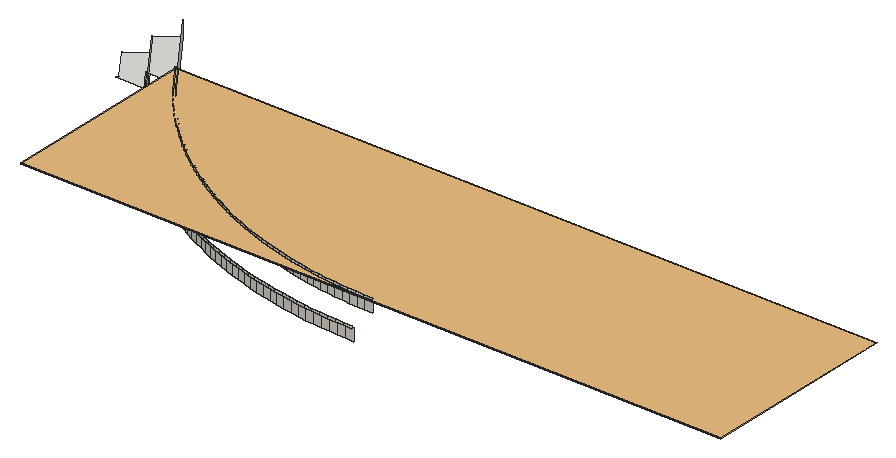
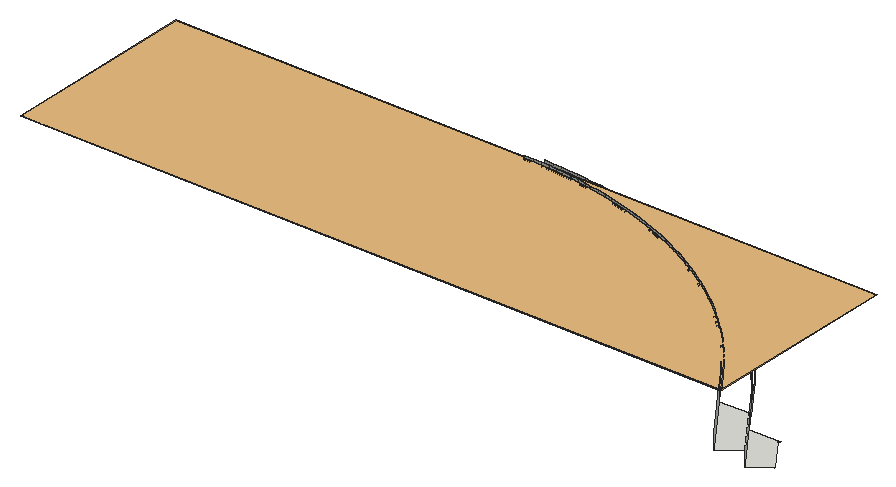
# SketchUp Ruby script. Lengths in inches.
U = 1.inch
M = Sketchup.active_model
def pt(a) = Geom::Point3d.new(a.map { |v| v * U })
def face(e, loops, mat)
  f = e.add_face(loops[0].map { |a| pt(a) })
  loops[1..].each { |l| e.add_face(l.map { |a| pt(a) }).erase! }
  f.material = f.back_material = mat if mat
  f
end
# faces: each face lists its corners as indices into pts; further lists are holes
def faces(e, pts, list, mat = nil) = list.each { |f| face(e, (f[0].is_a?(Array) ? f : [f]).map { |l| l.map { |i| pts[i] } }, mat) }
# xy, xz, yz: faces in a plane at the given z, y or x. An outline is a flat list of corners, or four numbers for a rectangle; further outlines are holes
def ring(l) = l.size == 4 ? [[l[0], l[1]], [l[2], l[1]], [l[2], l[3]], [l[0], l[3]]] : l.each_slice(2).to_a
def flat(e, list, mat, &to3) = list.each { |f| face(e, (f[0].is_a?(Array) ? f : [f]).map { |l| ring(l).map { |u, v| to3.(u, v) } }, mat) }
def xy(e, z, list, mat = nil) = flat(e, list, mat) { |x, y| [x, y, z] }
def xz(e, y, list, mat = nil) = flat(e, list, mat) { |x, z| [x, y, z] }
def yz(e, x, list, mat = nil) = flat(e, list, mat) { |y, z| [x, y, z] }
def lines(e, pts, list) = list.each { |a, b| e.add_line(pt(pts[a]), pt(pts[b])) }
# prism: a flat outline (further loops are holes) pulled along v
def prism(e, loops, v, mat = nil)
  f = face(e, loops, mat); d = Geom::Vector3d.new(v.map { |x| x * U })
  f.pushpull(f.normal.samedirection?(d) ? d.length : -d.length)
end
def box(e, o, s, mat = nil) = prism(e, [[o, [o[0] + s[0], o[1], o[2]], [o[0] + s[0], o[1] + s[1], o[2]], [o[0], o[1] + s[1], o[2]]]], [0, 0, s[2]], mat)
def at(x, y, z, deg = 0) = Geom::Transformation.translation(pt([x, y, z])) * Geom::Transformation.rotation(ORIGIN, Z_AXIS, deg.degrees)
def axes(o, x, y, z) = Geom::Transformation.new([*x, 0, *y, 0, *z, 0, *pt(o).to_a, 1])
def part(name) = M.definitions.add(name)
# library, detail: a bought-in or finely detailed component or shape, given as its bounding box
def library(name, o, s) = part(name).tap { |d| box(d.entities, o, s) }
def detail(e, o, s) = box(e.add_group.entities, o, s)
def put(e, d, t, mat = nil) = e.add_instance(d, t).tap { |i| i.material = mat if mat }
def group(e, t, mat = nil) = e.add_group.tap { |g| g.transformation = t; g.material = mat if mat }.entities
root = M.entities
M.materials.add("Arta-Ceramic-Moonstone-White-24x24-4K").color = [209, 205, 196]
c1 = library("Mesh Light\#5",[-0.5,-0.5,-0.1],[1,1,0.2])
xy(root,18,[[859.84,194.875,871.84,194.875,857.89,214.375,849.96,208.69,859.5,195.35]])
xy(root,18,[[858.84,194.875,859.84,194.875,859.5,195.35]],"Arta-Ceramic-Moonstone-White-24x24-4K")
xy(root,23,[[870.84,194.875,870.78,194.96,871.44,195.43,871.84,194.875]],"Arta-Ceramic-Moonstone-White-24x24-4K")
xy(root,24,[[871.84,194.875,883.84,194.875,865.83,220.05,857.89,214.375,871.44,195.43]])
xy(root,24,[[870.84,194.875,871.84,194.875,871.44,195.43,870.78,194.96]],"Arta-Ceramic-Moonstone-White-24x24-4K")
xy(root,29,[[882.84,194.875,882.57,195.26,883.23,195.73,883.84,194.875]],"Arta-Ceramic-Moonstone-White-24x24-4K")
p = [[1020.9,108.58,23],[1020.9,108.58,18],[1024.28,108.54,18],[1024.28,108.54,23],[1017.51,108.67,23],[1017.51,108.67,18],
  [1014.13,108.84,23],[1014.13,108.84,18],[1010.76,109.0625,23],[1010.76,109.0625,18],[1007.39,109.35,23],[1007.39,109.35,18],
  [1004.02,109.71,23],[1004.02,109.71,18],[1000.66,110.13,23],[1000.66,110.13,18],[997.3125,110.62,23],[997.3125,110.62,18],
  [993.97,111.17,23],[993.97,111.17,18],[990.65,111.78,23],[990.65,111.78,18],[987.33,112.46,23],[987.33,112.46,18],
  [984.03,113.2,23],[984.03,113.2,18],[980.74,114,23],[980.74,114,18],[977.47,114.87,23],[977.47,114.87,18],
  [974.22,115.8,23],[974.22,115.8,18],[970.98,116.79,23],[970.98,116.79,18],[967.77,117.84,23],[967.77,117.84,18],
  [964.57,118.96,23],[964.57,118.96,18],[961.4,120.13,23],[961.4,120.13,18],[958.25,121.37,23],[958.25,121.37,18],
  [955.12,122.67,23],[955.12,122.67,18],[952.02,124.02,23],[952.02,124.02,18],[948.95,125.44,23],[948.95,125.44,18],
  [945.9,126.92,23],[945.9,126.92,18],[942.88,128.45,23],[942.88,128.45,18],[939.9,130.04,23],[939.9,130.04,18],
  [936.94,131.6875,23],[936.94,131.6875,18],[934.02,133.39,23],[934.02,133.39,18],[931.13,135.15,23],[931.13,135.15,18],
  [928.27,136.96,23],[928.27,136.96,18],[925.45,138.83,23],[925.45,138.83,18],[922.67,140.76,23],[922.67,140.76,18],
  [919.92,142.73,23],[919.92,142.73,18],[917.21,144.76,23],[917.21,144.76,18],[914.54,146.84,23],[914.54,146.84,18],
  [911.91,148.97,23],[911.91,148.97,18],[909.32,151.15,23],[909.32,151.15,18],[906.78,153.38,23],[906.78,153.38,18],
  [904.28,155.66,23],[904.28,155.66,18],[901.82,157.99,23],[901.82,157.99,18],[899.41,160.36,23],[899.41,160.36,18],
  [897.04,162.78,23],[897.04,162.78,18],[894.72,165.24,23],[894.72,165.24,18],[892.45,167.75,23],[892.45,167.75,18],
  [890.22,170.3,23],[890.22,170.3,18],[888.05,172.89,23],[888.05,172.89,18],[885.92,175.53,23],[885.92,175.53,18],
  [883.85,178.2,23],[883.85,178.2,18],[881.83,180.92,23],[881.83,180.92,18],[871.84,194.875,23],[871.84,194.875,18],
  [857.89,214.375,18],[871.44,195.43,23],[871.44,195.43,24],[857.89,214.375,24],[1020.88,107.76,24],[1020.88,107.76,23],
  [1024.28,107.73,23],[1024.28,107.73,24],[1017.48,107.86,24],[1017.48,107.86,23],[1014.09,108.02,24],[1014.09,108.02,23],
  [1010.7,108.25,24],[1010.7,108.25,23],[1007.31,108.54,24],[1007.31,108.54,23],[1003.93,108.9,24],[1003.93,108.9,23],
  [1000.55,109.33,24],[1000.55,109.33,23],[997.19,109.8125,24],[997.19,109.8125,23],[993.84,110.37,24],[993.84,110.37,23],
  [990.49,110.98,24],[990.49,110.98,23],[987.16,111.66,24],[987.16,111.66,23],[983.84,112.41,24],[983.84,112.41,23],
  [980.54,113.21,24],[980.54,113.21,23],[977.25,114.08,24],[977.25,114.08,23],[973.99,115.02,24],[973.99,115.02,23],
  [970.74,116.01,24],[970.74,116.01,23],[967.5,117.07,24],[967.5,117.07,23],[964.29,118.19,24],[964.29,118.19,23],
  [961.11,119.375,24],[961.11,119.375,23],[957.94,120.62,24],[957.94,120.62,23],[954.8,121.92,24],[954.8,121.92,23],
  [951.6875,123.28,24],[951.6875,123.28,23],[948.6,124.71,24],[948.6,124.71,23],[945.54,126.1875,24],[945.54,126.1875,23],
  [942.51,127.73,24],[942.51,127.73,23],[939.51,129.32,24],[939.51,129.32,23],[936.54,130.98,24],[936.54,130.98,23],
  [933.6,132.69,24],[933.6,132.69,23],[930.7,134.46,24],[930.7,134.46,23],[927.83,136.28,24],[927.83,136.28,23],
  [924.99,138.16,24],[924.99,138.16,23],[922.2,140.09,24],[922.2,140.09,23],[919.4375,142.08,24],[919.4375,142.08,23],
  [916.72,144.11,24],[916.72,144.11,23],[914.03,146.2,24],[914.03,146.2,23],[911.39,148.34,24],[911.39,148.34,23],
  [908.79,150.54,24],[908.79,150.54,23],[906.24,152.78,24],[906.24,152.78,23],[903.72,155.07,24],[903.72,155.07,23],
  [901.25,157.4,24],[901.25,157.4,23],[898.83,159.79,24],[898.83,159.79,23],[896.45,162.22,24],[896.45,162.22,23],
  [894.12,164.69,24],[894.12,164.69,23],[891.84,167.21,24],[891.84,167.21,23],[889.61,169.77,24],[889.61,169.77,23],
  [887.42,172.38,24],[887.42,172.38,23],[885.29,175.02,24],[885.29,175.02,23],[883.2,177.71,24],[883.2,177.71,23],
  [881.17,180.4375,24],[881.17,180.4375,23],[870.84,194.875,24],[870.84,194.875,23],[870.78,194.96,23],[870.78,194.96,24],
  [1017.89,118.43,29],[1017.89,118.43,24],[1021.08,118.33,24],[1021.08,118.33,29],[1024.28,118.3,24],[1024.28,118.3,29],
  [1014.7,118.58,29],[1014.7,118.58,24],[1011.51,118.79,29],[1011.51,118.79,24],[1008.32,119.07,29],[1008.32,119.07,24],
  [1005.14,119.41,29],[1005.14,119.41,24],[1001.97,119.8,29],[1001.97,119.8,24],[998.81,120.26,29],[998.81,120.26,24],
  [995.65,120.78,29],[995.65,120.78,24],[992.51,121.36,29],[992.51,121.36,24],[989.375,122,29],[989.375,122,24],
  [986.26,122.7,29],[986.26,122.7,24],[983.15,123.46,29],[983.15,123.46,24],[980.0625,124.28,29],[980.0625,124.28,24],
  [976.99,125.16,29],[976.99,125.16,24],[973.93,126.09,29],[973.93,126.09,24],[970.89,127.09,29],[970.89,127.09,24],
  [967.875,128.14,29],[967.875,128.14,24],[964.875,129.25,29],[964.875,129.25,24],[961.9,130.42,29],[961.9,130.42,24],
  [958.95,131.65,29],[958.95,131.65,24],[956.02,132.93,29],[956.02,132.93,24],[953.12,134.27,29],[953.12,134.27,24],
  [950.24,135.66,29],[950.24,135.66,24],[947.39,137.11,29],[947.39,137.11,24],[944.57,138.61,29],[944.57,138.61,24],
  [941.77,140.16,29],[941.77,140.16,24],[939.01,141.77,29],[939.01,141.77,24],[936.28,143.4375,29],[936.28,143.4375,24],
  [933.58,145.15,29],[933.58,145.15,24],[930.92,146.92,29],[930.92,146.92,24],[928.29,148.73,29],[928.29,148.73,24],
  [925.69,150.6,29],[925.69,150.6,24],[923.13,152.52,29],[923.13,152.52,24],[920.61,154.48,29],[920.61,154.48,24],
  [918.13,156.49,29],[918.13,156.49,24],[915.68,158.55,29],[915.68,158.55,24],[913.28,160.66,29],[913.28,160.66,24],
  [910.92,162.8125,29],[910.92,162.8125,24],[908.59,165.01,29],[908.59,165.01,24],[906.32,167.25,29],[906.32,167.25,24],
  [904.08,169.54,29],[904.08,169.54,24],[901.89,171.87,29],[901.89,171.87,24],[899.74,174.23,29],[899.74,174.23,24],
  [897.64,176.64,29],[897.64,176.64,24],[895.59,179.09,29],[895.59,179.09,24],[893.58,181.58,29],[893.58,181.58,24],
  [891.62,184.11,29],[891.62,184.11,24],[889.71,186.67,29],[889.71,186.67,24],[883.84,194.875,29],[883.84,194.875,24],
  [865.83,220.05,24],[883.23,195.73,29],[883.23,195.73,30],[865.83,220.05,30],[1017.86,117.61,30],[1017.86,117.61,29],
  [1021.07,117.52,29],[1021.07,117.52,30],[1024.28,117.49,29],[1024.28,117.49,30],[1014.65,117.77,30],[1014.65,117.77,29],
  [1011.44,117.98,30],[1011.44,117.98,29],[1008.24,118.26,30],[1008.24,118.26,29],[1005.05,118.6,30],[1005.05,118.6,29],
  [1001.86,119,30],[1001.86,119,29],[998.68,119.46,30],[998.68,119.46,29],[995.51,119.98,30],[995.51,119.98,29],
  [992.35,120.5625,30],[992.35,120.5625,29],[989.21,121.2,30],[989.21,121.2,29],[986.07,121.91,30],[986.07,121.91,29],
  [982.95,122.67,30],[982.95,122.67,29],[979.85,123.49,30],[979.85,123.49,29],[976.76,124.375,30],[976.76,124.375,29],
  [973.68,125.32,30],[973.68,125.32,29],[970.63,126.32,30],[970.63,126.32,29],[967.6,127.375,30],[967.6,127.375,29],
  [964.59,128.49,30],[964.59,128.49,29],[961.6,129.67,30],[961.6,129.67,29],[958.63,130.9,30],[958.63,130.9,29],
  [955.6875,132.1875,30],[955.6875,132.1875,29],[952.77,133.53,30],[952.77,133.53,29],[949.88,134.93,30],[949.88,134.93,29],
  [947.01,136.38,30],[947.01,136.38,29],[944.18,137.89,30],[944.18,137.89,29],[941.37,139.46,30],[941.37,139.46,29],
  [938.6,141.08,30],[938.6,141.08,29],[935.85,142.75,30],[935.85,142.75,29],[933.14,144.47,30],[933.14,144.47,29],
  [930.46,146.24,30],[930.46,146.24,29],[927.82,148.07,30],[927.82,148.07,29],[925.21,149.94,30],[925.21,149.94,29],
  [922.64,151.87,30],[922.64,151.87,29],[920.11,153.84,30],[920.11,153.84,29],[917.61,155.87,30],[917.61,155.87,29],
  [915.15,157.9375,30],[915.15,157.9375,29],[912.74,160.05,30],[912.74,160.05,29],[910.36,162.22,30],[910.36,162.22,29],
  [908.03,164.43,30],[908.03,164.43,29],[905.74,166.68,30],[905.74,166.68,29],[903.49,168.97,30],[903.49,168.97,29],
  [901.29,171.3125,30],[901.29,171.3125,29],[899.13,173.69,30],[899.13,173.69,29],[897.02,176.12,30],[897.02,176.12,29],
  [894.96,178.58,30],[894.96,178.58,29],[892.94,181.08,30],[892.94,181.08,29],[890.97,183.62,30],[890.97,183.62,29],
  [889.06,186.19,30],[889.06,186.19,29],[882.84,194.875,30],[882.84,194.875,29],[882.57,195.26,29],[882.57,195.26,30]]
faces(root,p,[[0,1,2,3],[4,5,1,0],[6,7,5,4],[8,9,7,6],[10,11,9,8],[12,13,11,10],[14,15,13,12],[16,17,15,14],
  [18,19,17,16],[20,21,19,18],[22,23,21,20],[24,25,23,22],[26,27,25,24],[28,29,27,26],[30,31,29,28],[32,33,31,30],
  [34,35,33,32],[36,37,35,34],[38,39,37,36],[40,41,39,38],[42,43,41,40],[44,45,43,42],[46,47,45,44],[48,49,47,46],
  [50,51,49,48],[52,53,51,50],[54,55,53,52],[56,57,55,54],[58,59,57,56],[60,61,59,58],[62,63,61,60],[64,65,63,62],
  [66,67,65,64],[68,69,67,66],[70,71,69,68],[72,73,71,70],[74,75,73,72],[76,77,75,74],[78,79,77,76],[80,81,79,78],
  [82,83,81,80],[84,85,83,82],[86,87,85,84],[88,89,87,86],[90,91,89,88],[92,93,91,90],[94,95,93,92],[96,97,95,94],
  [98,99,97,96],[100,101,99,98],[106,107,108,109],[110,111,107,106],[112,113,111,110],[114,115,113,112],[116,117,115,114],[118,119,117,116],
  [120,121,119,118],[122,123,121,120],[124,125,123,122],[126,127,125,124],[128,129,127,126],[130,131,129,128],[132,133,131,130],[134,135,133,132],
  [136,137,135,134],[138,139,137,136],[140,141,139,138],[142,143,141,140],[144,145,143,142],[146,147,145,144],[148,149,147,146],[150,151,149,148],
  [152,153,151,150],[154,155,153,152],[156,157,155,154],[158,159,157,156],[160,161,159,158],[162,163,161,160],[164,165,163,162],[166,167,165,164],
  [168,169,167,166],[170,171,169,168],[172,173,171,170],[174,175,173,172],[176,177,175,174],[178,179,177,176],[180,181,179,178],[182,183,181,180],
  [184,185,183,182],[186,187,185,184],[188,189,187,186],[190,191,189,188],[192,193,191,190],[194,195,193,192],[196,197,195,194],[198,199,197,196],
  [200,201,199,198],[202,203,201,200],[204,205,203,202],[204,206,207,205],[208,207,206,209],[103,208,209,104],[210,211,212,213],[213,212,214,215],
  [216,217,211,210],[218,219,217,216],[220,221,219,218],[222,223,221,220],[224,225,223,222],[226,227,225,224],[228,229,227,226],[230,231,229,228],
  [232,233,231,230],[234,235,233,232],[236,237,235,234],[238,239,237,236],[240,241,239,238],[242,243,241,240],[244,245,243,242],[246,247,245,244],
  [248,249,247,246],[250,251,249,248],[252,253,251,250],[254,255,253,252],[256,257,255,254],[258,259,257,256],[260,261,259,258],[262,263,261,260],
  [264,265,263,262],[266,267,265,264],[268,269,267,266],[270,271,269,268],[272,273,271,270],[274,275,273,272],[276,277,275,274],[278,279,277,276],
  [280,281,279,278],[282,283,281,280],[284,285,283,282],[286,287,285,284],[288,289,287,286],[290,291,289,288],[292,293,291,290],[294,295,293,292],
  [296,297,295,294],[298,299,297,296],[300,301,299,298],[302,303,301,300],[304,305,303,302],[306,307,305,304],[308,309,307,306],[310,311,309,308],
  [316,317,318,319],[319,318,320,321],[322,323,317,316],[324,325,323,322],[326,327,325,324],[328,329,327,326],[330,331,329,328],[332,333,331,330],
  [334,335,333,332],[336,337,335,334],[338,339,337,336],[340,341,339,338],[342,343,341,340],[344,345,343,342],[346,347,345,344],[348,349,347,346],
  [350,351,349,348],[352,353,351,350],[354,355,353,352],[356,357,355,354],[358,359,357,356],[360,361,359,358],[362,363,361,360],[364,365,363,362],
  [366,367,365,364],[368,369,367,366],[370,371,369,368],[372,373,371,370],[374,375,373,372],[376,377,375,374],[378,379,377,376],[380,381,379,378],
  [382,383,381,380],[384,385,383,382],[386,387,385,384],[388,389,387,386],[390,391,389,388],[392,393,391,390],[394,395,393,392],[396,397,395,394],
  [398,399,397,396],[400,401,399,398],[402,403,401,400],[404,405,403,402],[406,407,405,404],[408,409,407,406],[410,411,409,408],[412,413,411,410],
  [414,415,413,412],[414,416,417,415],[418,417,416,419],[314,313,418,419]],"Arta-Ceramic-Moonstone-White-24x24-4K")
faces(root,p,[[102,101,100,103,104,105],[312,311,310,313,314,315]])
g1 = group(root,at(882.84,117.49,29))
xy(g1,0,[[141.4375,0,138.23,0.03,135.01,0.125,131.81,0.28,128.6,0.49,125.4,0.77,122.21,1.11,119.02,1.51,115.84,1.97,112.67,2.49,109.51,3.07,106.36,3.72,103.23,4.42,100.11,5.18,97,6,93.91,6.89,90.84,7.83,87.79,8.83,84.76,9.89,81.74,11,78.75,12.18,75.79,13.41,72.84,14.7,69.93,16.04,67.03,17.44,64.17,18.9,61.33,20.4,58.53,21.97,55.75,23.59,53.01,25.26,50.3,26.98,47.62,28.75,44.98,30.58,42.37,32.46,39.8,34.38,37.26,36.36,34.77,38.38,32.3125,40.45,29.9,42.57,27.52,44.73,25.1875,46.9375,22.9,49.1875,20.65,51.49,18.45,53.82,16.29,56.2,14.18,58.625,12.12,61.09,10.1,63.59,8.13,66.13,6.21,68.7,0,77.39,1,77.39,6.87,69.18,8.78,66.62,10.74,64.09,12.74,61.6,14.8,59.15,16.9,56.74,19.04,54.375,21.24,52.05,23.47,49.76,25.75,47.52,28.07,45.32,30.4375,43.17,32.84,41.07,35.29,39,37.77,36.99,40.29,35.03,42.85,33.11,45.44,31.24,48.08,29.43,50.74,27.66,53.4375,25.95,56.17,24.29,58.93,22.68,61.72,21.12,64.55,19.62,67.4,18.17,70.27,16.78,73.18,15.4375,76.11,14.16,79.06,12.93,82.03,11.76,85.03,10.65,88.05,9.6,91.09,8.6,94.14,7.67,97.22,6.79,100.31,5.97,103.41,5.21,106.53,4.51,109.66,3.87,112.81,3.29,115.96,2.77,119.125,2.3125,122.3,1.92,125.48,1.58,128.66,1.3,131.85,1.09,135.05,0.9375,138.24,0.84,141.4375,0.8125,144.63,0.84,147.83,0.9375,151.02,1.09,154.21,1.3,157.4,1.58,160.58,1.92,163.75,2.3125,166.91,2.77,170.07,3.29,173.21,3.87,176.34,4.51,179.46,5.21,182.57,5.97,185.66,6.79,188.73,7.67,191.79,8.6,194.83,9.6,197.84,10.65,200.84,11.76,203.82,12.93,206.77,14.16,209.7,15.4375,212.6,16.78,215.48,18.17,218.33,19.62,221.15,21.12,223.94,22.68,226.71,24.29,229.4375,25.95,232.13,27.66,234.8,29.43,237.43,31.24,240.03,33.11,242.58,35.03,245.11,36.99,247.59,39,250.03,41.07,252.4375,43.17,254.8,45.32,257.125,47.52,259.4,49.76,261.64,52.05,263.83,54.375,265.98,56.74,268.08,59.15,270.13,61.6,272.14,64.09,274.1,66.62,276.01,69.18,281.875,77.39,282.2,77.84,282.86,77.37,276.66,68.7,274.74,66.13,272.78,63.59,270.76,61.09,268.7,58.625,266.58,56.2,264.43,53.82,262.23,51.49,259.98,49.1875,257.6875,46.9375,255.35,44.73,252.98,42.57,250.5625,40.45,248.11,38.38,245.61,36.36,243.08,34.38,240.51,32.46,237.9,30.58,235.26,28.75,232.58,26.98,229.87,25.26,227.12,23.59,224.35,21.97,221.54,20.4,218.7,18.9,215.84,17.44,212.95,16.04,210.03,14.7,207.09,13.41,204.12,12.18,201.13,11,198.12,9.89,195.09,8.83,192.03,7.83,188.96,6.89,185.875,6,182.77,5.18,179.65,4.42,176.51,3.72,173.37,3.07,170.21,2.49,167.04,1.97,163.86,1.51,160.67,1.11,157.48,0.77,154.27,0.49,151.07,0.28,147.86,0.125,144.65,0.03]],"Arta-Ceramic-Moonstone-White-24x24-4K")
put(g1,c1,axes([141.43,38.92,0],[283.86372,0,0],[0,78.84297,0],[0,0,1]))
